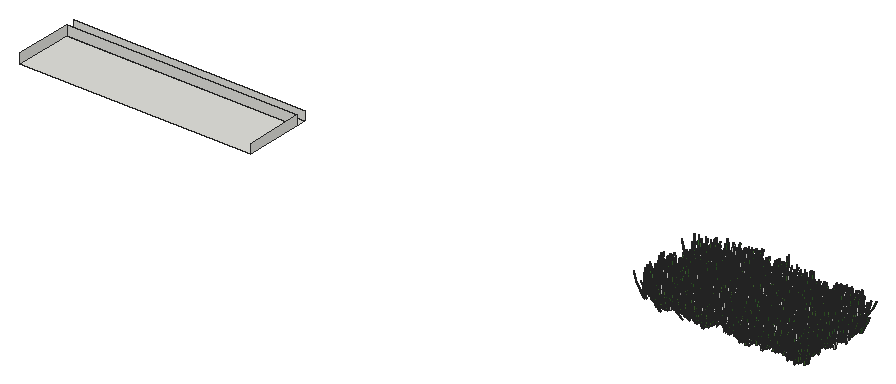
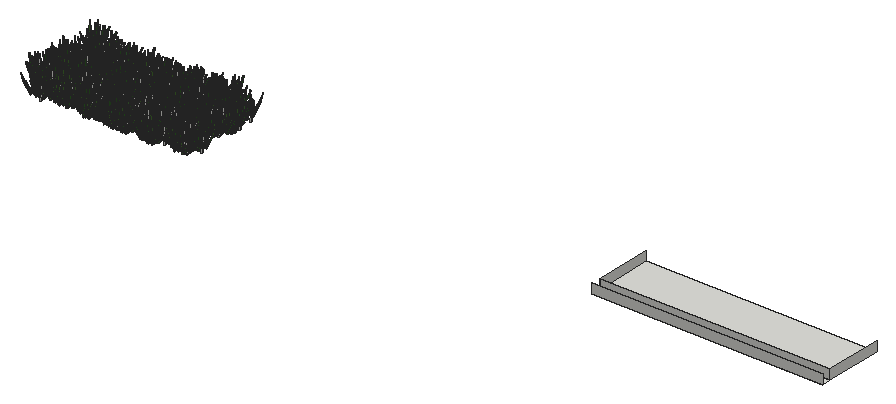
# SketchUp Ruby script. Lengths in inches.
U = 1.inch
M = Sketchup.active_model
def pt(a) = Geom::Point3d.new(a.map { |v| v * U })
def face(e, loops, mat)
  f = e.add_face(loops[0].map { |a| pt(a) })
  loops[1..].each { |l| e.add_face(l.map { |a| pt(a) }).erase! }
  f.material = f.back_material = mat if mat
  f
end
# faces: each face lists its corners as indices into pts; further lists are holes
def faces(e, pts, list, mat = nil) = list.each { |f| face(e, (f[0].is_a?(Array) ? f : [f]).map { |l| l.map { |i| pts[i] } }, mat) }
# xy, xz, yz: faces in a plane at the given z, y or x. An outline is a flat list of corners, or four numbers for a rectangle; further outlines are holes
def ring(l) = l.size == 4 ? [[l[0], l[1]], [l[2], l[1]], [l[2], l[3]], [l[0], l[3]]] : l.each_slice(2).to_a
def flat(e, list, mat, &to3) = list.each { |f| face(e, (f[0].is_a?(Array) ? f : [f]).map { |l| ring(l).map { |u, v| to3.(u, v) } }, mat) }
def xy(e, z, list, mat = nil) = flat(e, list, mat) { |x, y| [x, y, z] }
def xz(e, y, list, mat = nil) = flat(e, list, mat) { |x, z| [x, y, z] }
def yz(e, x, list, mat = nil) = flat(e, list, mat) { |y, z| [x, y, z] }
def lines(e, pts, list) = list.each { |a, b| e.add_line(pt(pts[a]), pt(pts[b])) }
# prism: a flat outline (further loops are holes) pulled along v
def prism(e, loops, v, mat = nil)
  f = face(e, loops, mat); d = Geom::Vector3d.new(v.map { |x| x * U })
  f.pushpull(f.normal.samedirection?(d) ? d.length : -d.length)
end
def box(e, o, s, mat = nil) = prism(e, [[o, [o[0] + s[0], o[1], o[2]], [o[0] + s[0], o[1] + s[1], o[2]], [o[0], o[1] + s[1], o[2]]]], [0, 0, s[2]], mat)
def at(x, y, z, deg = 0) = Geom::Transformation.translation(pt([x, y, z])) * Geom::Transformation.rotation(ORIGIN, Z_AXIS, deg.degrees)
def axes(o, x, y, z) = Geom::Transformation.new([*x, 0, *y, 0, *z, 0, *pt(o).to_a, 1])
def part(name) = M.definitions.add(name)
# library, detail: a bought-in or finely detailed component or shape, given as its bounding box
def library(name, o, s) = part(name).tap { |d| box(d.entities, o, s) }
def detail(e, o, s) = box(e.add_group.entities, o, s)
def put(e, d, t, mat = nil) = e.add_instance(d, t).tap { |i| i.material = mat if mat }
def group(e, t, mat = nil) = e.add_group.tap { |g| g.transformation = t; g.material = mat if mat }.entities
root = M.entities
M.materials.add("Material1").color = [58, 110, 58]
M.materials.add("Material10").color = [48, 100, 38]
M.materials.add("Material3").color = [68, 110, 58]
M.materials.add("Material4").color = [48, 90, 38]
M.materials.add("Material5").color = [68, 110, 48]
M.materials.add("Material6").color = [48, 90, 48]
M.materials.add("Material8").color = [58, 90, 38]
M.materials.add("Material9").color = [68, 100, 58]
c1 = part("Group\#69")
xy(c1.entities,0,[[0,0,48,2]])
c2 = part("grass00")
p = [[-0.6875,0.15,0],[-0.56,0.08,5.52],[-0.04,0.03,2.76],[0.48,-0.02,0],[0.35,-0.02,5.52],[-0.1,-0.14,5.52],
  [-0.12,0.65,8.37],[-0.42,0.65,8.37]]
faces(c2.entities,p,[[0,1,2,3],[3,2,4],[1,5,2],[5,4,2],[1,6,5],[4,5,6],[7,6,1]])
c3 = part("Group16\#1")
put(c3.entities,c2,axes([1.44,-0.61,-0.01],[0.05352,0.12609,0],[-0.10704,0.04543,0.07239],[0.06664,-0.02828,0.11628]),"Material6")
put(c3.entities,c2,axes([0.76,-0.15,-0.01],[0.04676,0.24062,0],[-0.23162,0.04501,0.06642],[0.0652,-0.01267,0.23595]),"Material3")
put(c3.entities,c2,axes([0.79,0.01,-0.01],[-0.00606,0.34651,0],[-0.34381,-0.00602,0.0432],[0.04319,0.00076,0.34386]))
put(c3.entities,c2,axes([1,0.23,-0.01],[-0.07192,0.31144,0],[-0.28722,-0.06632,0.1236],[0.12043,0.02781,0.29478]),"Material5")
put(c3.entities,c2,axes([1.66,0.77,-0.01],[-0.13828,0.29651,0],[-0.21551,-0.1005,0.22471],[0.20365,0.09498,0.23779]),"Material10")
put(c3.entities,c2,axes([0.6875,0.52,-0.01],[-0.18126,0.24051,0],[-0.22746,-0.17142,0.09788],[0.07817,0.05891,0.28481]),"Material5")
put(c3.entities,c2,axes([0.68,0.78,-0.01],[-0.215,0.18688,0],[-0.12385,-0.14248,0.21334],[0.13995,0.16101,0.18878]),"Material3")
put(c3.entities,c2,axes([0.56,1,-0.01],[-0.13756,0.07624,0],[-0.06159,-0.11112,0.0927],[0.04494,0.08108,0.12705]),"Material5")
put(c3.entities,c2,axes([0.2,0.64,-0.01],[-0.23729,0.07254,0],[-0.05711,-0.18681,0.153],[0.04473,0.14632,0.19535]),"Material10")
put(c3.entities,c2,axes([0.0625,0.72,-0.01],[-0.28874,0.02525,0],[-0.02179,-0.24916,0.14647],[0.01276,0.14591,0.25012]),"Material3")
put(c3.entities,c2,axes([-0.08,0.62,-0.01],[-0.34089,-0.04187,0],[0.03255,-0.26504,0.216],[-0.02633,0.21439,0.26703]),"Material10")
put(c3.entities,c2,axes([-0.34,0.98,-0.01],[-0.14314,-0.0493,0],[0.04397,-0.12769,0.06843],[-0.02228,0.0647,0.13505]),"Material10")
put(c3.entities,c2,axes([-0.87,1.45,-0.01],[-0.23488,-0.14114,0],[0.13761,-0.22901,0.06087],[-0.03135,0.05217,0.26717]))
put(c3.entities,c2,axes([-0.72,0.77,-0.01],[-0.14208,-0.13251,0],[0.07209,-0.0773,0.16301],[-0.11118,0.11922,0.1057]),"Material10")
put(c3.entities,c2,axes([-0.62,0.43,-0.01],[-0.14845,-0.21203,0],[0.18654,-0.13061,0.12304],[-0.10079,0.07057,0.22772]),"Material3")
put(c3.entities,c2,axes([-0.68,0.29,-0.01],[-0.13639,-0.32136,0],[0.31723,-0.13464,0.05579],[-0.05136,0.0218,0.34462]),"Material4")
put(c3.entities,c2,axes([-0.64,0.125,-0.01],[-0.0458,-0.23569,0],[0.22124,-0.043,0.08276],[-0.08124,0.01579,0.22538]),"Material1")
put(c3.entities,c2,axes([-1.6,-0.03,-0.01],[0.00576,-0.32897,0],[0.27526,0.00482,0.18018],[-0.18015,-0.00315,0.2753]),"Material5")
put(c3.entities,c2,axes([-1.36,-0.31,-0.01],[0.05718,-0.24765,0],[0.18172,0.04196,0.17267],[-0.16825,-0.03885,0.1865]),"Material10")
put(c3.entities,c2,axes([-1.54,-0.72,-0.01],[0.06537,-0.14017,0],[0.13555,0.06321,0.03939],[-0.0357,-0.01665,0.14956]))
put(c3.entities,c2,axes([-1.19,-0.9,-0.01],[0.09597,-0.12735,0],[0.11214,0.08451,0.07557],[-0.06035,-0.04548,0.14042]),"Material9")
put(c3.entities,c2,axes([-0.47,-0.54,-0.01],[0.11588,-0.10072,0],[0.0618,0.0711,0.12124],[-0.07953,-0.0915,0.0942]))
put(c3.entities,c2,axes([-0.47,-0.84,-0.01],[0.11927,-0.0661,0],[0.06603,0.11913,0.00646],[-0.00313,-0.00565,0.13621]),"Material5")
put(c3.entities,c2,axes([-0.38,-1.24,-0.01],[0.28037,-0.08571,0],[0.0618,0.20215,0.20315],[-0.05939,-0.19428,0.21139]),"Material9")
put(c3.entities,c2,axes([-0.06,-0.66,-0.01],[0.22719,-0.01987,0],[0.01247,0.14255,0.17758],[-0.01547,-0.17691,0.1431]),"Material8")
put(c3.entities,c2,axes([0.11,-0.89,-0.01],[0.14882,0.01828,0],[-0.01058,0.08611,0.12229],[0.01491,-0.12138,0.08676]),"Material6")
put(c3.entities,c2,axes([0.25,-0.72,-0.01],[0.20481,0.07053,0],[-0.06206,0.18022,0.10291],[0.03351,-0.0973,0.1906]),"Material6")
put(c3.entities,c2,axes([0.85,-1.42,-0.01],[0.16481,0.09904,0],[-0.09472,0.15762,0.05616],[0.02893,-0.04814,0.18389]),"Material5")
put(c3.entities,c2,axes([1.01,-1.09,-0.01],[0.21858,0.20385,0],[-0.17495,0.1876,0.15339],[0.10462,-0.11218,0.25652]),"Material10")
put(c3.entities,c2,axes([1.01,-0.71,-0.01],[0.08733,0.12473,0],[-0.06445,0.04512,0.13037],[0.1068,-0.07477,0.07867]),"Material6")
c4 = part("Group15\#1")
put(c4.entities,c3,at(0,0,0))
c5 = part("3darcstudiotree_grass00\#1")
put(c5.entities,c4,at(0,0,0))
xy(root,0,[[138.47,128.5,186.47,140.5]])
xz(root,140.5,[[138.47,0,186.47,2]])
xz(root,142.5,[[138.47,0,186.47,2]])
yz(root,138.47,[[128.5,0,140.5,2]])
yz(root,186.47,[[128.5,0,140.5,2]])
put(root,c1,at(138.47,140.5,0))
put(root,c5,axes([266.34,137.3,0.25],[-0.83802,-0.33874,0],[0.4564,-0.77783,-0.03924],[0.03181,-0.05422,1.93013]))
put(root,c5,axes([266.58,145.08,0.25],[0.91864,0.48015,0],[-0.55397,0.73015,-0.03908],[-0.03652,0.04813,1.82303]))
put(root,c5,axes([266.78,135.95,0.25],[0.78163,0.82293,0],[-0.76498,0.50055,-0.04305],[-0.05274,0.03451,1.51958]))
put(root,c5,axes([267.29,132.27,0.25],[0.86176,0.69503,0],[-0.85929,0.73397,-0.06236],[-0.06562,0.05605,1.86199]))
put(root,c5,axes([267.65,147,0.25],[0.33573,-0.70766,0],[1.03544,0.33841,-0.0431],[0.04981,0.01628,1.38217]))
put(root,c5,axes([267.67,139.54,0.25],[0.57447,-0.59174,0],[0.96717,0.64684,-0.04335],[0.04201,0.02809,1.54559]))
put(root,c5,axes([267.63,137.5,0.25],[-0.74591,0.71792,0],[-0.97262,-0.69616,-0.04683],[-0.05149,-0.03686,1.86493]))
put(root,c5,axes([267.9375,138.58,0.25],[0.19477,-0.76602,0],[1.18228,0.20709,-0.04294],[0.04667,0.00817,1.34209]))
put(root,c5,axes([268.11,143.82,0.25],[0.31078,-0.77045,0],[1.11807,0.3107,-0.04023],[0.04414,0.01227,1.36415]))
put(root,c5,axes([268.28,133.84,0.25],[0.70479,-0.63594,0],[0.83226,0.63542,-0.05921],[0.07395,0.05646,1.91907]))
put(root,c5,axes([268.89,137.34,0.25],[-1.20206,-0.39206,0],[0.40587,-0.85725,-0.03326],[0.01692,-0.03574,1.54402]))
put(root,c5,axes([269.74,139.96,0.25],[-1.07815,-0.43691,0],[0.56282,-0.95678,-0.06565],[0.03818,-0.06491,1.70067]))
put(root,c5,axes([269.77,138.03,0.25],[0.85847,-0.54829,0],[0.58482,0.6308,-0.03629],[0.03263,0.0352,1.41389]))
put(root,c5,axes([270.4,146,0.25],[0.28199,-0.89828,0],[0.94777,0.20497,-0.04641],[0.06755,0.01461,1.47323]))
put(root,c5,axes([270.73,141.02,0.25],[-1.13838,-0.00895,0],[0.01219,-1.06851,-0.04475],[0.00047,-0.04137,1.43393]))
put(root,c5,axes([271.1,130.92,0.25],[-0.45694,-0.96595,0],[1.05779,-0.34471,-0.05278],[0.0803,-0.02617,1.85719]))
put(root,c5,axes([271.13,131.79,0.25],[-1.19329,-0.08357,0],[0.10038,-0.98738,-0.02802],[0.00355,-0.03496,1.8014]))
put(root,c5,axes([270.77,138.27,0.25],[1.00243,0.00164,0],[-0.00181,0.76391,-0.0306],[-0.00012,0.0525,1.9022]))
put(root,c5,axes([270.88,136.26,0.25],[0.86492,0.66202,0],[-0.82195,0.73979,-0.03053],[-0.03344,0.0301,1.95907]))
put(root,c5,axes([271.98,142.08,0.25],[-0.96063,0.66845,0],[-0.73694,-0.72959,-0.04843],[-0.03848,-0.03809,1.41858]))
put(root,c5,axes([272.03,144.87,0.25],[0.72804,-0.79745,0],[0.84234,0.52978,-0.04967],[0.06509,0.04094,1.73743]))
put(root,c5,axes([271.86,134.48,0.25],[0.8851,0.49287,0],[-0.60001,0.74231,-0.0468],[-0.03887,0.04808,1.60535]))
put(root,c5,axes([272.11,145.74,0.25],[1.25572,-0.17259,0],[0.2107,1.05608,-0.06031],[0.01517,0.07604,1.9859]))
put(root,c5,axes([272.45,133.49,0.25],[0.13808,-0.92265,0],[1.04172,0.1074,-0.05019],[0.07262,0.00749,1.53052]))
put(root,c5,axes([272.26,143.84,0.25],[0.8896,0.2464,0],[-0.39241,0.97599,-0.04175],[-0.01621,0.04033,1.52086]))
put(root,c5,axes([272.36,135.6875,0.25],[1.12086,-0.13328,0],[0.12926,0.74887,-0.032],[0.00994,0.0576,1.99674]))
put(root,c5,axes([273.83,147.43,0.25],[0.06537,-0.89425,0],[1.19384,0.06012,-0.04584],[0.05029,0.00253,1.3146]))
put(root,c5,axes([273.96,140.21,0.25],[-0.20255,-0.83026,0],[1.02526,-0.17231,-0.04711],[0.06655,-0.01119,1.50792]))
put(root,c5,axes([273.76,131.93,0.25],[-0.26333,0.85426,0],[-1.01527,-0.2156,-0.04208],[-0.05991,-0.01272,1.54007]))
put(root,c5,axes([274.16,142.24,0.25],[-0.08829,-0.77336,0],[1.25458,-0.09867,-0.03587],[0.04546,-0.00358,1.60406]))
put(root,c5,axes([274,141.07,0.25],[1.01348,0.01813,0],[-0.02137,0.82266,-0.0399],[-0.00164,0.06298,1.8861]))
put(root,c5,axes([275.12,138.1875,0.25],[-1.28141,0.16443,0],[-0.14808,-0.79499,-0.03554],[-0.01029,-0.05524,1.83631]))
put(root,c5,axes([274.77,141.92,0.25],[-0.02824,0.89669,0],[-1.1218,-0.02434,-0.03889],[-0.0523,-0.00113,1.50954]))
put(root,c5,axes([275.43,147.14,0.25],[-0.32992,-0.73416,0],[1.08888,-0.3371,-0.0406],[0.06046,-0.01872,1.84742]))
put(root,c5,axes([275.1875,146.51,0.25],[0.53756,0.94912,0],[-0.97638,0.38096,-0.03464],[-0.05176,0.0202,1.78143]))
put(root,c5,axes([275.81,131,0.25],[-0.61937,-0.84339,0],[0.919,-0.46494,-0.05337],[0.06401,-0.03238,1.5119]))
put(root,c5,axes([275.68,143.27,0.25],[0.57666,-0.90262,0],[1.11576,0.49107,-0.05067],[0.05373,0.02365,1.51576]))
put(root,c5,axes([275.66,132.03,0.25],[0.57041,-0.92027,0],[0.86378,0.36883,-0.03693],[0.06,0.02562,1.77491]))
put(root,c5,axes([276.42,146.04,0.25],[-0.87935,0.73853,0],[-0.71119,-0.58335,-0.03007],[-0.04217,-0.03459,1.97134]))
put(root,c5,axes([276.625,143.14,0.25],[-0.46532,0.86414,0],[-0.89032,-0.33027,-0.0353],[-0.0592,-0.02196,1.79152]))
put(root,c5,axes([276.96,136.9,0.25],[-0.78813,-0.50794,0],[0.76881,-0.82179,-0.06125],[0.04078,-0.04359,1.36064]))
put(root,c5,axes([276.84,139.79,0.25],[0.03234,-1.06804,0],[1.07365,0.0224,-0.05528],[0.08224,0.00172,1.59813]))
put(root,c5,axes([277.2,138.57,0.25],[-0.59367,-0.81757,0],[0.79657,-0.39847,-0.03107],[0.04763,-0.02382,1.66455]))
put(root,c5,axes([277.29,130.93,0.25],[0.12126,-0.89919,0],[1.06781,0.0992,-0.04376],[0.06149,0.00571,1.51939]))
put(root,c5,axes([278.28,137.49,0.25],[0.61557,-0.59039,0],[0.89397,0.64212,-0.03846],[0.03885,0.02791,1.57923]))
put(root,c5,axes([278.58,136.11,0.25],[-0.59472,-0.84138,0],[0.93591,-0.45573,-0.03431],[0.04199,-0.02045,1.53951]))
put(root,c5,axes([278.4,143.43,0.25],[0.72186,-0.83935,0],[1.00266,0.59405,-0.04124],[0.04253,0.0252,1.56101]))
put(root,c5,axes([278.6875,145.78,0.25],[0.13948,-0.87163,0],[1.23109,0.13571,-0.03191],[0.04379,0.00483,1.71939]))
put(root,c5,axes([278.76,139.29,0.25],[-0.95782,-0.29691,0],[0.43507,-0.9669,-0.03885],[0.01949,-0.04331,1.78292]))
put(root,c5,axes([279.44,132.51,0.25],[-1.23455,-0.09168,0],[0.10565,-0.98012,-0.03473],[0.00448,-0.04155,1.7157]))
put(root,c5,axes([279.63,140.67,0.25],[-0.35323,-0.91476,0],[1.08057,-0.28745,-0.03893],[0.05368,-0.01428,1.64312]))
put(root,c5,axes([279.7,142.23,0.25],[-0.92328,-0.73148,0],[0.83739,-0.72814,-0.04863],[0.05418,-0.04711,1.95701]))
put(root,c5,axes([279.64,130.52,0.25],[-0.21916,-0.84158,0],[1.16712,-0.20938,-0.06129],[0.06711,-0.01204,1.3376]))
put(root,c5,axes([279.63,147.43,0.25],[0.19464,-0.82605,0],[1.26682,0.20564,-0.06032],[0.06469,0.0105,1.41053]))
put(root,c5,axes([280.34,144.9,0.25],[-1.03414,0.47897,0],[-0.5011,-0.74534,-0.03544],[-0.02615,-0.0389,1.55733]))
put(root,c5,axes([280.86,143.08,0.25],[-0.97453,-0.66212,0],[0.66069,-0.6699,-0.04086],[0.04363,-0.04424,1.75811]))
put(root,c5,axes([281.04,134.31,0.25],[-0.53982,-0.83264,0],[1.00723,-0.44986,-0.04084],[0.04976,-0.02222,1.58232]))
put(root,c5,axes([280.99,133.55,0.25],[-0.96182,0.06924,0],[-0.09601,-0.91873,-0.04163],[-0.00613,-0.05867,1.89396]))
put(root,c5,axes([281.1875,138.3,0.25],[0.82867,0.33155,0],[-0.40601,0.69908,-0.04063],[-0.0289,0.04977,1.53169]))
put(root,c5,axes([281.23,135.55,0.25],[-0.21653,0.79482,0],[-1.24807,-0.23423,-0.04071],[-0.04465,-0.00838,1.43871]))
put(root,c5,axes([281.86,147.17,0.25],[0.35241,-1.01641,0],[1.22375,0.2923,-0.04991],[0.07319,0.01748,1.94306]))
put(root,c5,axes([281.62,141.16,0.25],[1.00703,0.12031,0],[-0.15689,0.90468,-0.04848],[-0.00947,0.05462,1.51023]))
put(root,c5,axes([281.92,145.03,0.25],[0.49414,-0.90866,0],[1.1349,0.42517,-0.03311],[0.04629,0.01734,1.9099]))
put(root,c5,axes([282.48,146.86,0.25],[-0.52473,0.95642,0],[-0.82371,-0.31133,-0.04508],[-0.06009,-0.02271,1.32557]))
put(root,c5,axes([282.48,142.07,0.25],[1.08875,-0.05812,0],[0.08,1.03237,-0.04097],[0.00351,0.04527,1.66267]))
put(root,c5,axes([282.66,145.63,0.25],[0.81111,-0.54946,0],[0.60699,0.61728,-0.03627],[0.04512,0.04588,1.88825]))
put(root,c5,axes([282.98,137.05,0.25],[-0.72463,-0.78408,0],[0.83764,-0.53329,-0.03114],[0.04389,-0.02794,1.87535]))
put(root,c5,axes([282.58,138.74,0.25],[0.37438,0.73716,0],[-1.07212,0.3751,-0.04214],[-0.06462,0.02261,1.93625]))
put(root,c5,axes([283.21,132.23,0.25],[-1.07744,0.14364,0],[-0.17474,-0.90295,-0.04907],[-0.01154,-0.05965,1.63442]))
put(root,c5,axes([282.91,144.73,0.25],[0.24407,0.99771,0],[-1.24161,0.20925,-0.02679],[-0.03734,0.00629,1.80175]))
put(root,c5,axes([283.07,133.1875,0.25],[0.90252,-0.09445,0],[0.14465,0.95216,-0.05027],[0.00848,0.05582,1.55905]))
put(root,c5,axes([283.3,139.95,0.25],[0.8013,-0.42352,0],[0.52411,0.68313,-0.0345],[0.03513,0.04579,1.8497]))
put(root,c5,axes([283.93,142.58,0.25],[-0.72161,-0.73768,0],[0.96645,-0.65128,-0.02494],[0.03046,-0.02053,1.95866]))
put(root,c5,axes([284.16,143.89,0.25],[-0.78411,-0.37137,0],[0.49678,-0.72259,-0.04344],[0.04209,-0.06122,1.9596]))
put(root,c5,axes([284.23,136.91,0.25],[-0.45483,-0.87726,0],[1.12021,-0.40011,-0.04688],[0.05911,-0.02111,1.67419]))
put(root,c5,axes([284.64,139.71,0.25],[-0.42621,-0.9453,0],[1.18661,-0.36856,-0.05081],[0.05611,-0.01743,1.49393]))
put(root,c5,axes([284.78,133.13,0.25],[-1.07512,-0.09921,0],[0.12579,-0.93912,-0.05312],[0.00861,-0.0643,1.67036]))
put(root,c5,axes([284.64,131.15,0.25],[0.86017,0.22573,0],[-0.32245,0.84646,-0.04459],[-0.02097,0.05506,1.66873]))
put(root,c5,axes([284.89,134.9,0.25],[-0.58705,0.57695,0],[-0.8487,-0.59491,-0.03207],[-0.04391,-0.03078,1.99077]))
put(root,c5,axes([284.9375,136.06,0.25],[-0.83078,0.78387,0],[-0.96062,-0.70137,-0.06393],[-0.0527,-0.03848,1.40472]))
put(root,c5,axes([284.89,138.13,0.25],[1.24824,-0.09965,0],[0.12337,1.06455,-0.06081],[0.00654,0.0564,1.44654]))
put(root,c5,axes([285.4,146.92,0.25],[-0.01005,-0.7831,0],[1.28041,-0.01132,-0.05216],[0.05551,-0.00049,1.36288]))
put(root,c5,axes([285.54,140.84,0.25],[-1.02808,-0.65944,0],[0.7343,-0.78866,-0.06061],[0.04432,-0.04761,1.43628]))
put(root,c5,axes([285.47,145.76,0.25],[-0.9811,0.26517,0],[-0.29237,-0.74519,-0.04555],[-0.02405,-0.06129,1.60995]))
put(root,c5,axes([285.65,137.49,0.25],[-0.98394,0.6223,0],[-0.63093,-0.68723,-0.04347],[-0.0421,-0.04585,1.66314]))
put(root,c5,axes([286.16,142.06,0.25],[-1.10385,0.07367,0],[-0.0928,-0.95793,-0.04274],[-0.00388,-0.04001,1.31001]))
put(root,c5,axes([285.78,143.23,0.25],[0.68798,0.62687,0],[-0.89379,0.67576,-0.05824],[-0.05608,0.0424,1.57486]))
put(root,c5,axes([285.91,132.11,0.25],[0.7062,0.46844,0],[-0.60091,0.62408,-0.04441],[-0.05105,0.05302,1.772]))
put(root,c5,axes([287.11,143.52,0.25],[-0.45759,0.75389,0],[-0.94787,-0.39634,-0.03585],[-0.04785,-0.02001,1.58646]))
put(root,c5,axes([287.27,147.32,0.25],[-0.95842,0.54277,0],[-0.59226,-0.72046,-0.04776],[-0.04285,-0.05212,1.6727]))
put(root,c5,axes([287.65,146.12,0.25],[0.33108,-0.90959,0],[1.12278,0.28154,-0.03916],[0.05797,0.01454,1.81408]))
put(root,c5,axes([287.51,134.26,0.25],[0.90162,0.4573,0],[-0.65357,0.88772,-0.04231],[-0.03382,0.04594,1.92144]))
put(root,c5,axes([287.98,137.44,0.25],[-1.18579,0.1082,0],[-0.10184,-0.76887,-0.04038],[-0.00755,-0.05703,1.5952]))
put(root,c5,axes([288.51,138.77,0.25],[0.42146,-0.67797,0],[1.02979,0.44101,-0.04957],[0.06563,0.02811,1.72633]))
put(root,c5,axes([288.5625,137.36,0.25],[0.52352,-0.97358,0],[1.09625,0.40609,-0.04062],[0.05531,0.02049,1.79015]))
put(root,c5,axes([288.53,141.28,0.25],[0.86135,-0.26576,0],[0.37274,0.83223,-0.02775],[0.01739,0.03883,1.92398]))
put(root,c5,axes([288.6,130.13,0.25],[-0.27129,0.75081,0],[-0.88559,-0.22044,-0.04553],[-0.06155,-0.01532,1.30482]))
put(root,c5,axes([288.91,146.26,0.25],[-0.16262,-0.8641,0],[1.00766,-0.13064,-0.04759],[0.06221,-0.00807,1.34947]))
put(root,c5,axes([289.16,130.86,0.25],[1.20384,0.30206,0],[-0.27636,0.75877,-0.04581],[-0.02185,0.05999,1.57403]))
put(root,c5,axes([289.44,144.38,0.25],[1.18621,-0.19983,0],[0.21312,0.87149,-0.04034],[0.01368,0.05593,1.82611]))
put(root,c5,axes([290.09,144.86,0.25],[-1.22444,-0.24899,0],[0.30786,-1.04297,-0.038],[0.01323,-0.04483,1.89315]))
put(root,c5,axes([290.39,141.03,0.25],[0.66295,-0.68617,0],[0.89916,0.59847,-0.04277],[0.04641,0.03089,1.60323]))
put(root,c5,axes([290.65,134.83,0.25],[-1.23339,-0.07761,0],[0.09295,-1.01759,-0.05601],[0.00479,-0.05245,1.39118]))
put(root,c5,axes([290.6875,137.23,0.25],[-0.8369,-0.69133,0],[0.8215,-0.68509,-0.05331],[0.05546,-0.04625,1.71744]))
put(root,c5,axes([290.29,133.16,0.25],[0.25731,1.04739,0],[-1.12621,0.1906,-0.03996],[-0.04823,0.00816,1.416]))
put(root,c5,axes([290.66,145.9375,0.25],[-0.52489,0.75703,0],[-1.10491,-0.52776,-0.03664],[-0.03298,-0.01575,1.3241]))
put(root,c5,axes([290.72,142.19,0.25],[1.20169,-0.26495,0],[0.32324,1.00999,-0.06211],[0.02029,0.06339,1.60192]))
put(root,c5,axes([290.81,143.42,0.25],[1.14414,0.48881,0],[-0.55458,0.89425,-0.04224],[-0.02528,0.04076,1.58426]))
put(root,c5,axes([291.46,141.25,0.25],[-1.0918,0.45537,0],[-0.45192,-0.74644,-0.0516],[-0.04482,-0.07402,1.94674]))
put(root,c5,axes([291.6,143.51,0.25],[-1.05055,0.08055,0],[-0.08729,-0.7843,-0.04806],[-0.00739,-0.06643,1.58689]))
put(root,c5,axes([291.83,136.8,0.25],[-0.93616,0.091,0],[-0.11097,-0.78643,-0.03745],[-0.00687,-0.0487,1.50509]))
put(root,c5,axes([292.01,131.04,0.25],[-1.13709,0.50981,0],[-0.56764,-0.87221,-0.03525],[-0.01835,-0.0282,1.3087]))
put(root,c5,axes([291.73,142.37,0.25],[1.1452,0.47478,0],[-0.5128,0.85209,-0.04234],[-0.02367,0.03933,1.4356]))
put(root,c5,axes([292.52,146.84,0.25],[-1.16243,-0.11856,0],[0.14487,-0.97846,-0.04768],[0.00733,-0.04953,1.49744]))
put(root,c5,axes([292.11,138.33,0.25],[0.24099,0.87984,0],[-1.20278,0.22695,-0.06457],[-0.0738,0.01392,1.44574]))
put(root,c5,axes([292.39,132.1,0.25],[0.75051,-0.71097,0],[0.90759,0.66001,-0.04981],[0.05188,0.03773,1.67091]))
put(root,c5,axes([292.38,135.51,0.25],[0.43596,0.69579,0],[-0.9431,0.40708,-0.03549],[-0.04523,0.01952,1.52707]))
put(root,c5,axes([293.05,144.55,0.25],[-0.0133,-0.76852,0],[1.2506,-0.01491,-0.06189],[0.08257,-0.00098,1.66883]))
put(root,c5,axes([293.43,139.5625,0.25],[0.68838,-0.75988,0],[1.03488,0.64585,-0.05965],[0.07274,0.0454,1.97549]))
put(root,c5,axes([293.21,137.16,0.25],[1.22531,0.10986,0],[-0.13847,1.0639,-0.03307],[-0.00439,0.03373,1.59331]))
put(root,c5,axes([293.33,146.09,0.25],[0.15954,1.01492,0],[-0.9255,0.10022,-0.03746],[-0.06701,0.00726,1.68385]))
put(root,c5,axes([293.57,138.17,0.25],[0.67459,-0.80483,0],[0.78028,0.45054,-0.02795],[0.04495,0.02596,1.86246]))
put(root,c5,axes([293.87,134.7,0.25],[0.73371,-0.81835,0],[0.9838,0.60765,-0.05496],[0.05088,0.03143,1.41537]))
put(root,c5,axes([294.52,144.6,0.25],[0.36512,-0.78851,0],[0.96948,0.30926,-0.03841],[0.06038,0.01926,1.74904]))
put(root,c5,axes([294.78,131.39,0.25],[-0.71524,0.71441,0],[-0.75493,-0.52068,-0.04997],[-0.05749,-0.03965,1.46822]))
put(root,c5,axes([294.87,139.65,0.25],[1.14213,-0.04532,0],[0.04359,0.75677,-0.03217],[0.00292,0.05065,1.73328]))
put(root,c5,axes([294.98,146.49,0.25],[0.8951,0.40342,0],[-0.4567,0.69808,-0.03457],[-0.03314,0.05065,1.92264]))
put(root,c5,axes([296.09,133.4,0.25],[-0.09563,-1.04336,0],[1.26843,-0.08009,-0.05882],[0.07374,-0.00466,1.5994]))
put(root,c5,axes([296.22,145.875,0.25],[-0.48481,0.66427,0],[-1.09021,-0.54813,-0.05645],[-0.075,-0.03771,1.97994]))
put(root,c5,axes([296.18,144.91,0.25],[0.81562,0.50109,0],[-0.65207,0.73118,-0.05487],[-0.04319,0.04842,1.44987]))
put(root,c5,axes([296.52,143.66,0.25],[0.92111,-0.58078,0],[0.6014,0.65709,-0.03309],[0.02903,0.03172,1.44206]))
put(root,c5,axes([296.91,137.1,0.25],[-0.97924,-0.63232,0],[0.77963,-0.83175,-0.06227],[0.04131,-0.04407,1.37168]))
put(root,c5,axes([296.91,147.24,0.25],[1.09642,-0.06996,0],[0.0891,0.96199,-0.03486],[0.00387,0.04182,1.68524]))
put(root,c5,axes([297.8125,138.5625,0.25],[-1.00793,-0.20867,0],[0.23825,-0.79279,-0.04204],[0.01681,-0.05592,1.62585]))
put(root,c5,axes([297.72,130.85,0.25],[-1.03884,0.64597,0],[-0.69965,-0.77513,-0.03017],[-0.02678,-0.02966,1.72726]))
put(root,c5,axes([297.88,143.35,0.25],[0.90699,-0.31764,0],[0.49449,0.97269,-0.0407],[0.01883,0.03703,1.51351]))
put(root,c5,axes([297.91,139.7,0.25],[0.04122,0.75742,0],[-1.01346,0.038,-0.0329],[-0.06423,0.00241,1.98251]))
put(root,c5,axes([297.9,135.15,0.25],[-0.18804,0.98966,0],[-1.18673,-0.15533,-0.03641],[-0.0435,-0.00569,1.45326]))
put(root,c5,axes([298.45,137.17,0.25],[0.76984,0.50405,0],[-0.77843,0.81903,-0.06164],[-0.04106,0.0432,1.3518]))
put(root,c5,axes([298.54,133.33,0.25],[0.1317,0.88247,0],[-1.23544,0.12701,-0.03401],[-0.03809,0.00392,1.40523]))
put(root,c5,axes([299.22,143.07,0.25],[-1.00093,0.04601,0],[-0.05989,-0.89753,-0.04105],[-0.00384,-0.05756,1.83253]))
put(root,c5,axes([299.22,130.51,0.25],[-0.86318,0.40008,0],[-0.53161,-0.79014,-0.05669],[-0.04725,-0.07023,1.86391]))
put(root,c5,axes([299.39,137.18,0.25],[-0.64718,-0.75289,0],[0.78964,-0.46761,-0.04134],[0.06741,-0.03992,1.943]))
put(root,c5,axes([299.36,144.71,0.25],[0.77753,-0.82132,0],[0.87035,0.56761,-0.04001],[0.05218,0.03403,1.83572]))
put(root,c5,axes([299.17,141.11,0.25],[1.12461,0.26029,0],[-0.26308,0.78304,-0.03867],[-0.01862,0.05543,1.75619]))
put(root,c5,axes([299.71,139.95,0.25],[-0.82815,-0.67229,0],[0.7668,-0.65072,-0.0483],[0.04884,-0.04144,1.58573]))
